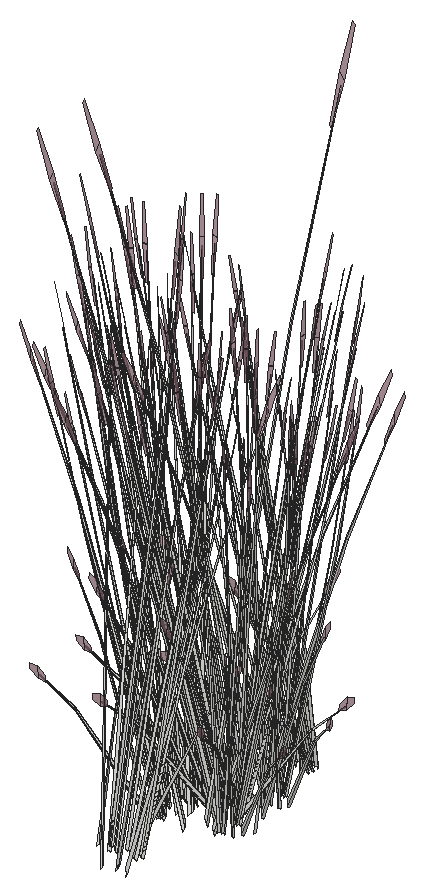
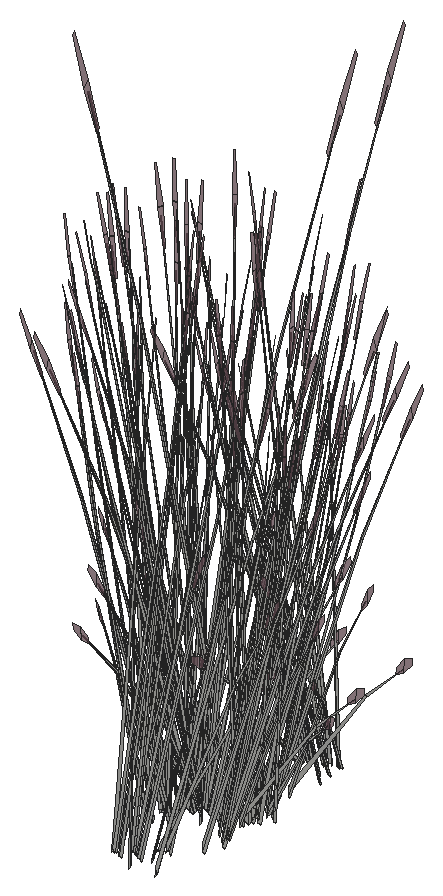
# SketchUp Ruby script. Lengths in inches.
U = 1.inch
M = Sketchup.active_model
def pt(a) = Geom::Point3d.new(a.map { |v| v * U })
def face(e, loops, mat)
  f = e.add_face(loops[0].map { |a| pt(a) })
  loops[1..].each { |l| e.add_face(l.map { |a| pt(a) }).erase! }
  f.material = f.back_material = mat if mat
  f
end
# faces: each face lists its corners as indices into pts; further lists are holes
def faces(e, pts, list, mat = nil) = list.each { |f| face(e, (f[0].is_a?(Array) ? f : [f]).map { |l| l.map { |i| pts[i] } }, mat) }
# xy, xz, yz: faces in a plane at the given z, y or x. An outline is a flat list of corners, or four numbers for a rectangle; further outlines are holes
def ring(l) = l.size == 4 ? [[l[0], l[1]], [l[2], l[1]], [l[2], l[3]], [l[0], l[3]]] : l.each_slice(2).to_a
def flat(e, list, mat, &to3) = list.each { |f| face(e, (f[0].is_a?(Array) ? f : [f]).map { |l| ring(l).map { |u, v| to3.(u, v) } }, mat) }
def xy(e, z, list, mat = nil) = flat(e, list, mat) { |x, y| [x, y, z] }
def xz(e, y, list, mat = nil) = flat(e, list, mat) { |x, z| [x, y, z] }
def yz(e, x, list, mat = nil) = flat(e, list, mat) { |y, z| [x, y, z] }
def lines(e, pts, list) = list.each { |a, b| e.add_line(pt(pts[a]), pt(pts[b])) }
# prism: a flat outline (further loops are holes) pulled along v
def prism(e, loops, v, mat = nil)
  f = face(e, loops, mat); d = Geom::Vector3d.new(v.map { |x| x * U })
  f.pushpull(f.normal.samedirection?(d) ? d.length : -d.length)
end
def box(e, o, s, mat = nil) = prism(e, [[o, [o[0] + s[0], o[1], o[2]], [o[0] + s[0], o[1] + s[1], o[2]], [o[0], o[1] + s[1], o[2]]]], [0, 0, s[2]], mat)
def at(x, y, z, deg = 0) = Geom::Transformation.translation(pt([x, y, z])) * Geom::Transformation.rotation(ORIGIN, Z_AXIS, deg.degrees)
def axes(o, x, y, z) = Geom::Transformation.new([*x, 0, *y, 0, *z, 0, *pt(o).to_a, 1])
def part(name) = M.definitions.add(name)
# library, detail: a bought-in or finely detailed component or shape, given as its bounding box
def library(name, o, s) = part(name).tap { |d| box(d.entities, o, s) }
def detail(e, o, s) = box(e.add_group.entities, o, s)
def put(e, d, t, mat = nil) = e.add_instance(d, t).tap { |i| i.material = mat if mat }
def group(e, t, mat = nil) = e.add_group.tap { |g| g.transformation = t; g.material = mat if mat }.entities
root = M.entities
M.materials.add("LightPink_Translucent").color = [144, 107, 117]
M.materials["LightPink_Translucent"].alpha = 0.75
c1 = part("blade")
p = [[2.15,0.21,22],[0,0.17,0],[0.09,0.45,0],[2.18,0.31,22],[2.29,0.31,22],[0.38,0.45,0],
  [2.48,0.24,33],[2.49,0.24,33],[2.48,0.22,33]]
faces(c1.entities,p,[[0,1,2,3],[4,5,2,3],[6,3,4,7],[8,0,3,6]])
c2 = part("seeds")
p = [[0.3,-0.1,1.38],[-0.01,-0.03,1.59],[-0.01,-0.03,0.03],[0.14,-0.07,-0.07],[0.29,-0.03,3],[0.15,0.01,3.11]]
faces(c2.entities,p,[[0,1,2,3],[1,0,4,5]],"LightPink_Translucent")
c3 = part("blade with seeds")
put(c3.entities,c1,at(0,0,0))
put(c3.entities,c2,axes([2.4,0.25,30.99],[1.5799,-0.05474,1.17369],[-0.12525,1.92788,0.29478],[-0.07173,-0.02425,1.56792]))
put(root,c3,axes([427.54,438.68,153.98],[-0.08817,-0.00333,1.47793],[-0.28072,0.33293,-0.23373],[-0.14978,-0.06803,0.11853]))
put(root,c3,axes([430.875,440.33,154.25],[-0.37908,-0.26007,-0.10273],[0.21839,-0.37663,-0.57019],[0.1071,-0.13092,0.8664]))
put(root,c3,axes([429.31,441.75,152.81],[0.35414,0.19019,1.27785],[-0.34693,0.40974,0.50532],[-0.1554,-0.24285,1.07126]))
put(root,c3,axes([429.7,435.65,154],[-0.18625,0.29962,0.05432],[-0.26523,-0.17444,0.42765],[0.08575,0.09606,0.65209]))
put(root,c3,axes([431.81,440.22,153.98],[-0.05353,-0.00358,1.49853],[-0.22227,-0.38383,-0.1416],[0.08926,-0.1262,0.26519]))
put(root,c3,axes([429.78,435.56,154],[-0.4076,0.10824,0.40553],[-0.07074,-0.4246,0.33437],[0.09586,0.12514,0.83914]))
put(root,c3,axes([427.77,434.39,153.27],[0.0763,-0.16212,1.44779],[0.3201,0.3355,0.11706],[-0.1444,0.2091,0.61892]))
put(root,c3,axes([430.98,440.07,153.82],[0.35672,-0.06741,-0.29918],[0.09419,0.38534,0.38624],[0.10222,-0.1035,0.73904]))
put(root,c3,axes([428.66,435.69,154],[-0.30197,0.1603,0.05432],[-0.1478,-0.29231,0.42765],[0.02916,0.12885,0.65209]))
put(root,c3,axes([427.85,435.31,153.82],[-0.27728,0.24833,-0.29918],[-0.26248,-0.28355,0.38624],[-0.03994,0.14407,0.73904]))
put(root,c3,axes([426.9,435.23,153.98],[-0.01019,0.09334,1.47793],[0.28908,0.3247,-0.23373],[-0.07568,0.15355,0.11853]))
put(root,c3,axes([427.63,439.43,154],[0.02064,-0.35866,0.05432],[0.3116,0.00983,0.42765],[-0.11936,-0.03753,0.65209]))
put(root,c3,axes([427.82,435.02,154.56],[0.45039,0.02337,-0.11403],[-0.01231,0.44247,-0.63292],[-0.03129,0.17041,0.9617]))
put(root,c3,axes([428.66,435.52,154.25],[0.40102,-0.2196,-0.10273],[0.19707,0.38974,-0.57019],[0.05291,0.16424,0.8664]))
put(root,c3,axes([427.51,439.54,153.82],[-0.23317,-0.29531,-0.29918],[0.26625,-0.27955,0.38624],[-0.13527,-0.04253,0.73904]))
put(root,c3,axes([428.2,442.64,153.27],[0.09368,0.15143,1.44779],[-0.43286,0.12749,0.11706],[-0.09783,-0.23774,0.61892]))
put(root,c3,axes([428.13,435.19,154.23],[0.29336,0.31691,-0.47917],[-0.3099,0.27755,-0.37115],[-0.04464,0.16102,0.91684]))
put(root,c3,axes([428.91,441.64,153.98],[-0.06268,-0.06613,1.47793],[-0.4183,0.04193,-0.23373],[-0.06676,-0.15817,0.11853]))
put(root,c3,axes([429,435.5,153.95],[0.40284,0.11824,-0.43168],[-0.13808,0.40538,-0.33437],[0.03694,0.16321,0.82598]))
put(root,c3,axes([429.23,434.66,153.27],[-0.09368,-0.15143,1.44779],[0.43286,-0.12749,0.11706],[0.09783,0.23774,0.61892]))
put(root,c3,axes([428.82,435.75,153.82],[-0.12355,0.36271,-0.29918],[-0.36044,-0.10579,0.38624],[0.03305,0.14603,0.73904]))
put(root,c3,axes([431.01,440.24,154],[0.28133,0.19836,0.05432],[-0.16379,0.28248,0.42765],[0.0902,-0.09132,0.65209]))
put(root,c3,axes([430.93,440.15,154],[0.10163,0.43409,0.40553],[-0.39868,0.07534,0.33437],[0.1175,-0.10209,0.83914]))
put(root,c3,axes([432.01,440.68,153.98],[0.05687,-0.07184,1.47793],[-0.07279,-0.44069,-0.23373],[0.14268,-0.08356,0.11853]))
put(root,c3,axes([428.04,435.05,154.51],[-0.01066,0.43628,-0.66621],[-0.44902,-0.0293,0.0804],[-0.04739,0.18483,0.94242]))
put(root,c3,axes([426.87,436.19,153.98],[0.04649,-0.02848,1.49853],[0.38427,0.18941,-0.1416],[-0.00903,0.15771,0.26519]))
put(root,c3,axes([427.2,438.96,153.98],[0.03038,0.04707,1.49853],[-0.14646,0.42312,-0.1416],[-0.14833,0.00306,0.26519]))
put(root,c3,axes([428.46,434.74,153.27],[-0.01003,-0.18103,1.44779],[0.43473,0.12009,0.11706],[-0.02689,0.25798,0.61892]))
put(root,c3,axes([430.79,442.45,153.98],[-0.00396,-0.09387,1.47793],[-0.33411,-0.2713,-0.23373],[0.05166,-0.16446,0.11853]))
put(root,c3,axes([429.39,442.43,153.82],[0.12355,-0.36271,-0.29918],[0.36044,0.10579,0.38624],[-0.03305,-0.14603,0.73904]))
put(root,c3,axes([429.66,442.91,153.27],[-0.0763,0.16212,1.44779],[-0.3201,-0.3355,0.11706],[0.1444,-0.2091,0.61892]))
put(root,c3,axes([430.7,442.11,153.98],[-0.04162,0.03603,1.49853],[-0.40776,-0.12155,-0.1416],[-0.01476,-0.15722,0.26519]))
put(root,c3,axes([427.625,439.83,153.95],[-0.29757,0.31243,-0.43168],[-0.2606,-0.33005,-0.33437],[-0.15119,-0.04754,0.82598]))
put(root,c3,axes([429.21,442.68,153.95],[-0.40284,-0.11824,-0.43168],[0.13808,-0.40538,-0.33437],[-0.03694,-0.16321,0.82598]))
put(root,c3,axes([428.5625,436.39,153.98],[0.05195,0.07595,1.47793],[0.41921,0.02984,-0.23373],[0.04216,0.1675,0.11853]))
put(root,c3,axes([430.08,442.99,153.95],[-0.29336,-0.31691,-0.43168],[0.3099,-0.27755,-0.33437],[0.04464,-0.16102,0.82598]))
put(root,c3,axes([427.78,439.51,154.25],[-0.02194,0.47967,-0.10273],[-0.41546,-0.01311,-0.57019],[-0.16001,-0.03332,0.8664]))
put(root,c3,axes([428.49,441.42,153.98],[-0.00765,0.05653,1.49853],[-0.37706,0.20517,-0.1416],[-0.11096,-0.10488,0.26519]))
put(root,c3,axes([430.89,441.35,154.25],[-0.20619,-0.42709,-0.10273],[0.36595,-0.20988,-0.57019],[0.15422,-0.05635,0.8664]))
put(root,c3,axes([430.87,440.98,153.95],[0.11102,-0.42903,-0.43168],[0.38064,0.14706,-0.33437],[0.15325,-0.03934,0.82598]))
put(root,c3,axes([427.25,440.17,153.27],[0.16998,-0.01068,1.44779],[-0.11276,0.46299,0.11706],[-0.24224,-0.02864,0.61892]))
put(root,c3,axes([429.43,442.51,154],[0.4038,0.12331,0.40553],[-0.13808,0.40538,0.33437],[-0.02427,-0.15942,0.83914]))
put(root,c3,axes([429.55,442.66,154.25],[-0.40102,0.2196,-0.10273],[-0.19707,-0.38974,-0.57019],[-0.05291,-0.16424,0.8664]))
put(root,c3,axes([430.38,443.15,154.25],[-0.45039,-0.02337,-0.10273],[0.01231,-0.44247,-0.57019],[0.03129,-0.17041,0.8664]))
put(root,c3,axes([430.35,442.87,153.82],[0.27728,-0.24833,-0.29918],[0.26248,0.28355,0.38624],[0.03994,-0.14407,0.73904]))
put(root,c3,axes([429.54,442.48,154],[0.30197,-0.1603,0.05432],[0.1478,0.29231,0.42765],[-0.02916,-0.12885,0.65209]))
put(root,c3,axes([428.35,442.5625,153.82],[-0.06329,-0.37991,-0.29918],[0.36182,-0.10032,0.38624],[-0.09718,-0.10887,0.73904]))
put(root,c3,axes([427.89,435.66,152.84],[0.009,-0.24349,1.30391],[0.40497,0.12861,0.18019],[-0.03509,0.2595,0.61571]))
put(root,c3,axes([428.51,442.53,154],[0.18625,-0.29962,0.05432],[0.26523,0.17444,0.42765],[-0.08575,-0.09606,0.65209]))
put(root,c3,axes([427.18,440.52,154],[0.11578,-0.43006,0.40553],[0.38064,0.14706,0.33437],[-0.14969,0.02584,0.83914]))
put(root,c3,axes([427.15,440.4,154],[-0.15051,-0.3216,0.05432],[0.27447,-0.15741,0.42765],[-0.12099,0.03106,0.65209]))
put(root,c3,axes([427.57,443.11,153.27],[0.15222,0.08126,1.44779],[-0.31502,0.34091,0.11706],[-0.19634,-0.15379,0.61892]))
put(root,c3,axes([428.31,442.875,153.95],[-0.40438,0.11212,-0.43168],[-0.07074,-0.4246,-0.33437],[-0.10862,-0.12168,0.82598]))
put(root,c3,axes([430.35,442.96,154],[0.29182,0.32181,0.40553],[-0.3099,0.27755,0.33437],[0.05383,-0.15098,0.83914]))
put(root,c3,axes([428.59,442.5,154.59],[-0.2735,0.45217,-0.11506],[-0.39608,-0.2605,-0.63862],[-0.13768,-0.12775,0.97037]))
put(root,c3,axes([430.46,443,154],[0.33677,0.02198,0.05432],[-0.00923,0.33185,0.42765],[0.03524,-0.12712,0.65209]))
put(root,c3,axes([431.1,441.18,153.82],[0.34057,0.13158,-0.29918],[-0.09933,0.38387,0.38624],[0.13712,-0.0352,0.73904]))
put(root,c3,axes([427.1,440.5625,153.82],[-0.34057,-0.13158,-0.29918],[0.09933,-0.38387,0.38624],[-0.13712,0.0352,0.73904]))
put(root,c3,axes([430.6875,443.72,153.95],[-0.10528,-0.43067,-0.43168],[0.39868,-0.07534,-0.33437],[0.11425,-0.11568,0.82598]))
put(root,c3,axes([430.18,440.7,153.27],[-0.16998,0.01068,1.44779],[0.11276,-0.46299,0.11706],[0.24224,0.02864,0.61892]))
put(root,c3,axes([427.54,442.37,153.98],[-0.08817,-0.00333,1.47793],[-0.28072,0.33293,-0.23373],[-0.14978,-0.06803,0.11853]))
put(root,c3,axes([430.875,444.02,154.25],[-0.37908,-0.26007,-0.10273],[0.21839,-0.37663,-0.57019],[0.1071,-0.13092,0.8664]))
put(root,c3,axes([431.05,441.34,154],[0.15051,0.3216,0.05432],[-0.27447,0.15741,0.42765],[0.12099,-0.03106,0.65209]))
put(root,c3,axes([431.03,441.22,154],[-0.11578,0.43006,0.40553],[-0.38064,-0.14706,0.33437],[0.14969,-0.02584,0.83914]))
put(root,c3,axes([429.31,445.44,152.81],[0.35414,0.19019,1.27785],[-0.34693,0.40974,0.50532],[-0.1554,-0.24285,1.07126]))
put(root,c3,axes([431.81,443.91,153.98],[-0.05353,-0.00358,1.49853],[-0.22227,-0.38383,-0.1416],[0.08926,-0.1262,0.26519]))
put(root,c3,axes([428.14,440.5,152.82],[0.11649,-0.06823,1.49584],[0.04017,0.47639,0.11706],[-0.25231,0.06321,0.53462]))
put(root,c3,axes([430.98,443.76,153.82],[0.35672,-0.06741,-0.29918],[0.09419,0.38534,0.38624],[0.10222,-0.1035,0.73904]))
put(root,c3,axes([427.63,443.12,154],[0.02064,-0.35866,0.05432],[0.3116,0.00983,0.42765],[-0.11936,-0.03753,0.65209]))
put(root,c3,axes([431.71,442.62,153.98],[-0.03706,-0.04129,1.49853],[0.08106,-0.44261,-0.1416],[0.14596,-0.02828,0.26519]))
put(root,c3,axes([427.51,443.23,153.82],[-0.23317,-0.29531,-0.29918],[0.26625,-0.27955,0.38624],[-0.13527,-0.04253,0.73904]))
put(root,c3,axes([426.89,440.82,153.98],[-0.06692,0.06124,1.47793],[0.00569,0.44742,-0.23373],[-0.15339,0.05818,0.11853]))
put(root,c3,axes([427.34,440.76,153.95],[-0.11102,0.42903,-0.43168],[-0.38064,-0.14706,-0.33437],[-0.15325,0.03934,0.82598]))
put(root,c3,axes([427.32,440.39,154.25],[0.20619,0.42709,-0.10273],[-0.36595,0.20988,-0.57019],[-0.15422,0.05635,0.8664]))
put(root,c3,axes([431.39,442.25,153.32],[-0.07843,-0.39649,-0.0295],[0.37072,-0.09115,-0.13375],[0.07742,0.02514,0.44114]))
put(root,c3,axes([430.43,442.23,154.25],[0.02194,-0.47967,-0.10273],[0.41546,0.01311,-0.57019],[0.16001,0.03332,0.8664]))
put(root,c3,axes([431.01,443.93,154],[0.28133,0.19836,0.05432],[-0.16379,0.28248,0.42765],[0.0902,-0.09132,0.65209]))
put(root,c3,axes([430.93,443.84,154],[0.10163,0.43409,0.40553],[-0.39868,0.07534,0.33437],[0.1175,-0.10209,0.83914]))
put(root,c3,axes([432.01,444.37,153.98],[0.05687,-0.07184,1.47793],[-0.07279,-0.44069,-0.23373],[0.14268,-0.08356,0.11853]))
put(root,c3,axes([430.79,441.95,153.98],[0.08791,-0.00798,1.47793],[0.24113,-0.36643,-0.23373],[0.15637,0.04837,0.11853]))
put(root,c3,axes([427.27,441.59,154],[-0.10163,-0.43409,0.40553],[0.39868,-0.07534,0.33437],[-0.1175,0.10209,0.83914]))
put(root,c3,axes([427.19,441.5,154],[-0.28133,-0.19836,0.05432],[0.16379,-0.28248,0.42765],[-0.0902,0.09132,0.65209]))
put(root,c3,axes([427.32,440.98,153.27],[0.14219,-0.09977,1.44779],[0.11971,0.461,0.11706],[-0.22323,0.10419,0.61892]))
put(root,c3,axes([427.2,442.65,153.98],[0.03038,0.04707,1.49853],[-0.14646,0.42312,-0.1416],[-0.14833,0.00306,0.26519]))
put(root,c3,axes([427.625,443.52,153.95],[-0.29757,0.31243,-0.43168],[-0.2606,-0.33005,-0.33437],[-0.15119,-0.04754,0.82598]))
put(root,c3,axes([427.78,443.2,154.25],[-0.02194,0.47967,-0.10273],[-0.41546,-0.01311,-0.57019],[-0.16001,-0.03332,0.8664]))
put(root,c3,axes([426.14,441.27,153.98],[0.0523,0.01265,1.49853],[0.16179,0.41674,-0.1416],[-0.10706,0.10938,0.26519]))
put(root,c3,axes([430.89,445.04,154.25],[-0.20619,-0.42709,-0.10273],[0.36595,-0.20988,-0.57019],[0.15422,-0.05635,0.8664]))
put(root,c3,axes([430.87,444.67,153.95],[0.11102,-0.42903,-0.43168],[0.38064,0.14706,-0.33437],[0.15325,-0.03934,0.82598]))
put(root,c3,axes([427.25,443.86,153.27],[0.16998,-0.01068,1.44779],[-0.11276,0.46299,0.11706],[-0.24224,-0.02864,0.61892]))
put(root,c3,axes([430.69,442.2,153.82],[0.23317,0.29531,-0.29918],[-0.26625,0.27955,0.38624],[0.13527,0.04253,0.73904]))
put(root,c3,axes([430.57,442.3125,154],[-0.02064,0.35866,0.05432],[-0.3116,-0.00983,0.42765],[0.11936,0.03753,0.65209]))
put(root,c3,axes([427.23,441.67,153.82],[-0.35672,0.06741,-0.29918],[-0.09419,-0.38534,0.38624],[-0.10222,0.1035,0.73904]))
put(root,c3,axes([430.6,442.2,154],[-0.30217,0.31079,0.40553],[-0.2606,-0.33005,0.33437],[0.14177,0.05733,0.83914]))
put(root,c3,axes([428.2,448.06,153.27],[0.09368,0.15143,1.44779],[-0.43286,0.12749,0.11706],[-0.09783,-0.23774,0.61892]))
put(root,c3,axes([429.86,441.44,153.27],[-0.15222,-0.08126,1.44779],[0.31502,-0.34091,0.11706],[0.19634,0.15379,0.61892]))
put(root,c3,axes([427.18,444.21,154],[0.11578,-0.43006,0.40553],[0.38064,0.14706,0.33437],[-0.14969,0.02584,0.83914]))
put(root,c3,axes([429.88,440.375,153.78],[-0.35411,-0.24507,1.16821],[0.37391,-0.38156,0.50405],[0.11425,0.22994,1.12919]))
put(root,c3,axes([428.91,447.0625,153.98],[-0.06268,-0.06613,1.47793],[-0.4183,0.04193,-0.23373],[-0.06676,-0.15817,0.11853]))
put(root,c3,axes([427.15,444.09,154],[-0.15051,-0.3216,0.05432],[0.27447,-0.15741,0.42765],[-0.12099,0.03106,0.65209]))
put(root,c3,axes([427.33,441.41,154.25],[0.37908,0.26007,-0.10273],[-0.21839,0.37663,-0.57019],[-0.1071,0.13092,0.8664]))
put(root,c3,axes([429.61,442.76,154.25],[0.2442,-0.40372,-0.10273],[0.35364,0.23259,-0.57019],[0.12293,0.11406,0.8664]))
put(root,c3,axes([427.84,441.29,153.27],[0.10236,-0.14492,1.44779],[0.25844,0.39118,0.11706],[-0.17726,0.17814,0.61892]))
put(root,c3,axes([427.52,441.72,153.95],[0.10528,0.43067,-0.43168],[-0.39868,0.07534,-0.33437],[-0.11425,0.11568,0.82598]))
put(root,c3,axes([431.1,444.87,153.82],[0.34057,0.13158,-0.29918],[-0.09933,0.38387,0.38624],[0.13712,-0.0352,0.73904]))
put(root,c3,axes([429.29,443.09,153.98],[0.00121,-0.0571,1.49853],[0.35119,-0.25193,-0.1416],[0.12199,0.08992,0.26519]))
put(root,c3,axes([427.1,444.26,153.82],[-0.34057,-0.13158,-0.29918],[0.09933,-0.38387,0.38624],[-0.13712,0.0352,0.73904]))
put(root,c3,axes([427.75,442.4375,154],[-0.33677,-0.02198,0.05432],[0.00923,-0.33185,0.42765],[-0.03524,0.12712,0.65209]))
put(root,c3,axes([427.85,442.47,154],[-0.29182,-0.32181,0.40553],[0.3099,-0.27755,0.33437],[-0.05383,0.15098,0.83914]))
put(root,c3,axes([429.9,442.56,153.95],[0.40438,-0.11212,-0.43168],[0.07074,0.4246,-0.33437],[0.10862,0.12168,0.82598]))
put(root,c3,axes([430.79,447.87,153.98],[-0.00396,-0.09387,1.47793],[-0.33411,-0.2713,-0.23373],[0.05166,-0.16446,0.11853]))
put(root,c3,axes([429.39,447.85,153.82],[0.12355,-0.36271,-0.29918],[0.36044,0.10579,0.38624],[-0.03305,-0.14603,0.73904]))
put(root,c3,axes([429.66,448.33,153.27],[-0.0763,0.16212,1.44779],[-0.3201,-0.3355,0.11706],[0.1444,-0.2091,0.61892]))
put(root,c3,axes([430.7,447.53,153.98],[-0.04162,0.03603,1.49853],[-0.40776,-0.12155,-0.1416],[-0.01476,-0.15722,0.26519]))
put(root,c3,axes([430.18,444.39,153.27],[-0.16998,0.01068,1.44779],[0.11276,-0.46299,0.11706],[0.24224,0.02864,0.61892]))
put(root,c3,axes([429.21,448.1,153.95],[-0.40284,-0.11824,-0.43168],[0.13808,-0.40538,-0.33437],[-0.03694,-0.16321,0.82598]))
put(root,c3,axes([431.05,445.03,154],[0.15051,0.3216,0.05432],[-0.27447,0.15741,0.42765],[0.12099,-0.03106,0.65209]))
put(root,c3,axes([430.08,448.41,153.95],[-0.29336,-0.31691,-0.43168],[0.3099,-0.27755,-0.33437],[0.04464,-0.16102,0.82598]))
put(root,c3,axes([431.03,444.91,154],[-0.11578,0.43006,0.40553],[-0.38064,-0.14706,0.33437],[0.14969,-0.02584,0.83914]))
put(root,c3,axes([429.7,442.9,154],[-0.18625,0.29962,0.05432],[-0.26523,-0.17444,0.42765],[0.08575,0.09606,0.65209]))
put(root,c3,axes([428.49,446.84,153.98],[-0.00765,0.05653,1.49853],[-0.37706,0.20517,-0.1416],[-0.11096,-0.10488,0.26519]))
put(root,c3,axes([429.78,442.82,154],[-0.4076,0.10824,0.40553],[-0.07074,-0.4246,0.33437],[0.09586,0.12514,0.83914]))
put(root,c3,axes([427.77,441.65,153.27],[0.0763,-0.16212,1.44779],[0.3201,0.3355,0.11706],[-0.1444,0.2091,0.61892]))
put(root,c3,axes([429.43,447.9375,154],[0.4038,0.12331,0.40553],[-0.13808,0.40538,0.33437],[-0.02427,-0.15942,0.83914]))
put(root,c3,axes([428.14,444.19,152.82],[0.11649,-0.06823,1.49584],[0.04017,0.47639,0.11706],[-0.25231,0.06321,0.53462]))
put(root,c3,axes([429.55,448.08,154.25],[-0.40102,0.2196,-0.10273],[-0.19707,-0.38974,-0.57019],[-0.05291,-0.16424,0.8664]))
put(root,c3,axes([430.38,448.57,154.25],[-0.45039,-0.02337,-0.10273],[0.01231,-0.44247,-0.57019],[0.03129,-0.17041,0.8664]))
put(root,c3,axes([430.35,448.29,153.82],[0.27728,-0.24833,-0.29918],[0.26248,0.28355,0.38624],[0.03994,-0.14407,0.73904]))
put(root,c3,axes([429.54,447.91,154],[0.30197,-0.1603,0.05432],[0.1478,0.29231,0.42765],[-0.02916,-0.12885,0.65209]))
put(root,c3,axes([428.35,447.98,153.82],[-0.06329,-0.37991,-0.29918],[0.36182,-0.10032,0.38624],[-0.09718,-0.10887,0.73904]))
